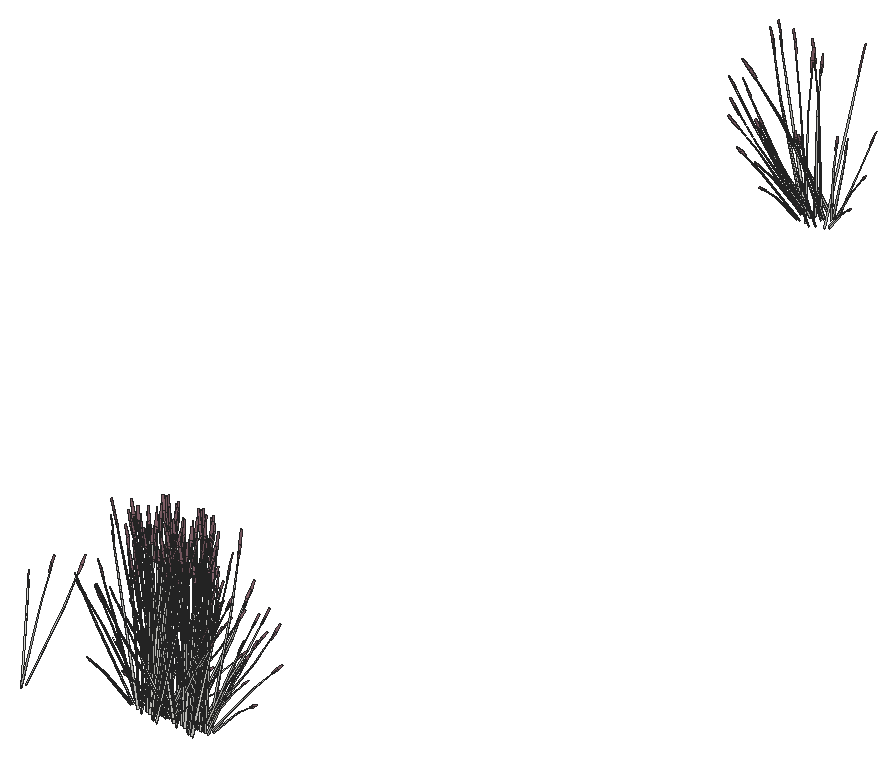
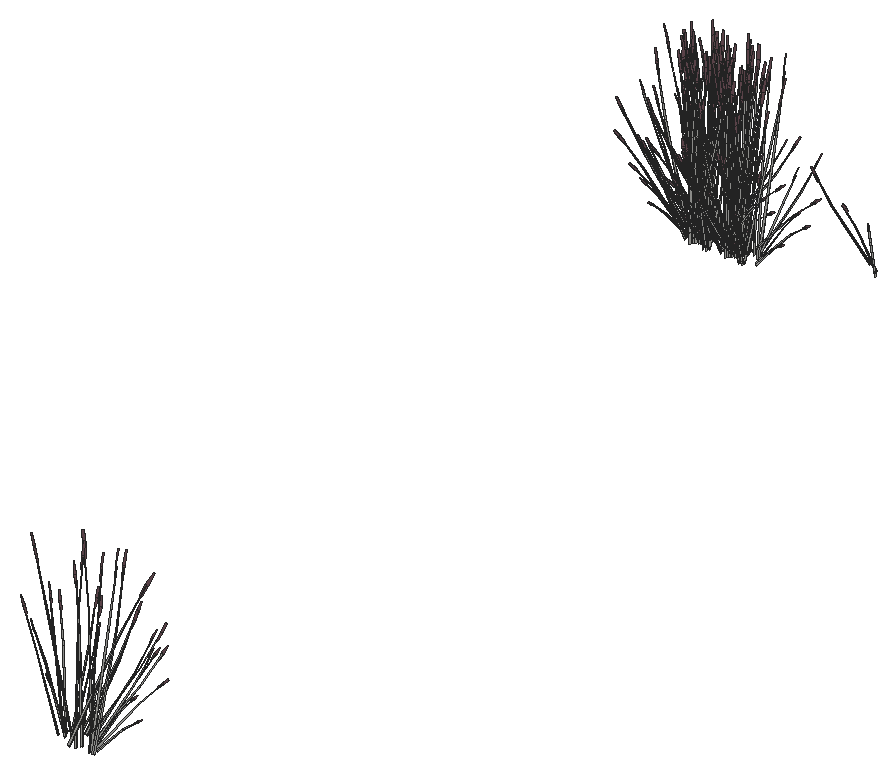
# SketchUp Ruby script. Lengths in inches.
U = 1.inch
M = Sketchup.active_model
def pt(a) = Geom::Point3d.new(a.map { |v| v * U })
def face(e, loops, mat)
  f = e.add_face(loops[0].map { |a| pt(a) })
  loops[1..].each { |l| e.add_face(l.map { |a| pt(a) }).erase! }
  f.material = f.back_material = mat if mat
  f
end
# faces: each face lists its corners as indices into pts; further lists are holes
def faces(e, pts, list, mat = nil) = list.each { |f| face(e, (f[0].is_a?(Array) ? f : [f]).map { |l| l.map { |i| pts[i] } }, mat) }
# xy, xz, yz: faces in a plane at the given z, y or x. An outline is a flat list of corners, or four numbers for a rectangle; further outlines are holes
def ring(l) = l.size == 4 ? [[l[0], l[1]], [l[2], l[1]], [l[2], l[3]], [l[0], l[3]]] : l.each_slice(2).to_a
def flat(e, list, mat, &to3) = list.each { |f| face(e, (f[0].is_a?(Array) ? f : [f]).map { |l| ring(l).map { |u, v| to3.(u, v) } }, mat) }
def xy(e, z, list, mat = nil) = flat(e, list, mat) { |x, y| [x, y, z] }
def xz(e, y, list, mat = nil) = flat(e, list, mat) { |x, z| [x, y, z] }
def yz(e, x, list, mat = nil) = flat(e, list, mat) { |y, z| [x, y, z] }
def lines(e, pts, list) = list.each { |a, b| e.add_line(pt(pts[a]), pt(pts[b])) }
# prism: a flat outline (further loops are holes) pulled along v
def prism(e, loops, v, mat = nil)
  f = face(e, loops, mat); d = Geom::Vector3d.new(v.map { |x| x * U })
  f.pushpull(f.normal.samedirection?(d) ? d.length : -d.length)
end
def box(e, o, s, mat = nil) = prism(e, [[o, [o[0] + s[0], o[1], o[2]], [o[0] + s[0], o[1] + s[1], o[2]], [o[0], o[1] + s[1], o[2]]]], [0, 0, s[2]], mat)
def at(x, y, z, deg = 0) = Geom::Transformation.translation(pt([x, y, z])) * Geom::Transformation.rotation(ORIGIN, Z_AXIS, deg.degrees)
def axes(o, x, y, z) = Geom::Transformation.new([*x, 0, *y, 0, *z, 0, *pt(o).to_a, 1])
def part(name) = M.definitions.add(name)
# library, detail: a bought-in or finely detailed component or shape, given as its bounding box
def library(name, o, s) = part(name).tap { |d| box(d.entities, o, s) }
def detail(e, o, s) = box(e.add_group.entities, o, s)
def put(e, d, t, mat = nil) = e.add_instance(d, t).tap { |i| i.material = mat if mat }
def group(e, t, mat = nil) = e.add_group.tap { |g| g.transformation = t; g.material = mat if mat }.entities
root = M.entities
M.materials.add("LightPink_Translucent").color = [144, 107, 117]
c1 = part("blade")
p = [[2.15,0.21,22],[0,0.17,0],[0.09,0.45,0],[2.18,0.31,22],[2.29,0.31,22],[0.38,0.45,0],
  [2.48,0.24,33],[2.49,0.24,33],[2.48,0.22,33]]
faces(c1.entities,p,[[0,1,2,3],[4,5,2,3],[6,3,4,7],[8,0,3,6]])
c2 = part("seeds")
p = [[0.3,-0.1,1.38],[-0.01,-0.03,1.59],[-0.01,-0.03,0.03],[0.14,-0.07,-0.07],[0.29,-0.03,3],[0.15,0.01,3.11]]
faces(c2.entities,p,[[0,1,2,3],[1,0,4,5]],"LightPink_Translucent")
c3 = part("blade with seeds")
put(c3.entities,c1,at(0,0,0))
put(c3.entities,c2,axes([2.4,0.25,30.99],[1.5799,-0.05474,1.17369],[-0.12525,1.92788,0.29478],[-0.07173,-0.02425,1.56792]))
put(root,c3,axes([71.27,71.75,46.98],[-1.22504,-0.02494,-0.71045],[0.08228,-1.05005,0.08574],[-0.51899,-0.11081,1.00501]))
put(root,c3,axes([30.98,61.23,46.98],[0.5849,0.8421,-0.71045],[-1.20401,0.4693,0.08574],[0.13677,0.40688,1.00501]))
put(root,c3,axes([27.6,62.55,44.59],[0.38672,-0.16338,1.43002],[0.95481,0.49262,-0.30754],[-0.28419,0.42626,0.61141]))
put(root,c3,axes([59.21,73.76,44.33],[-1.1399,0.87071,0.30756],[-1.1406,-0.86155,-0.36492],[-0.03981,-0.24727,1.64885]))
put(root,c3,axes([71.21,73.76,44.33],[-1.1399,0.87071,0.30756],[-1.1406,-0.86155,-0.36492],[-0.03981,-0.24727,1.64885]))
put(root,c3,axes([62.84,74.17,44.43],[1.3808,0.50196,0.24065],[-0.66454,1.04299,0.50002],[0,-0.24043,1.60543]))
put(root,c3,axes([74.84,74.17,44.43],[1.3808,0.50196,0.24065],[-0.66454,1.04299,0.50002],[0,-0.24043,1.60543]))
put(root,c3,axes([58.87,71.96,46.68],[-0.88986,0.68603,-0.51099],[-0.77932,-0.72471,-0.3958],[-0.45212,-0.10438,0.97773]))
put(root,c3,axes([70.87,71.96,46.68],[-0.88986,0.68603,-0.51099],[-0.77932,-0.72471,-0.3958],[-0.45212,-0.10438,0.97773]))
put(root,c3,axes([56.86,72.87,44.77],[0.78239,-0.07411,1.1486],[-0.49629,0.65296,0.84392],[-0.38663,-0.09795,0.25299]))
put(root,c3,axes([68.86,72.87,44.77],[0.78239,-0.07411,1.1486],[-0.49629,0.65296,0.84392],[-0.38663,-0.09795,0.25299]))
put(root,c3,axes([28.1,61.75,45.36],[0.02693,-0.53464,1.54345],[1.21102,0.2824,0.21329],[-0.10493,0.5698,0.72882]))
put(root,c3,axes([62.39,73.47,44.72],[-1.33077,0.06393,0.44739],[-0.12035,-1.06125,-0.21531],[0.23824,-0.10756,1.43643]))
put(root,c3,axes([74.39,73.47,44.72],[-1.33077,0.06393,0.44739],[-0.12035,-1.06125,-0.21531],[0.23824,-0.10756,1.43643]))
put(root,c3,axes([58.95,74.25,44.48],[0,1.03566,0.49651],[-1.37109,0,0],[0,-0.23588,1.57504]))
put(root,c3,axes([70.95,74.25,44.48],[0,1.03566,0.49651],[-1.37109,0,0],[0,-0.23588,1.57504]))
put(root,c3,axes([68.58,74.48,46.68],[0.332,-0.94205,-0.51099],[1.13828,0.3229,-0.3958],[0.45829,-0.08638,0.97773]))
put(root,c3,axes([80.58,74.48,46.68],[0.332,-0.94205,-0.51099],[1.13828,0.3229,-0.3958],[0.45829,-0.08638,0.97773]))
put(root,c3,axes([66.78,70.64,44.375],[0.7662,-1.03778,0],[1.28187,0.57875,-0.51607],[0.29196,0.13181,1.63711]))
put(root,c3,axes([78.78,70.64,44.375],[0.7662,-1.03778,0],[1.28187,0.57875,-0.51607],[0.29196,0.13181,1.63711]))
put(root,c3,axes([62.34,73.85,44.36],[0.53281,1.15808,0.45755],[-1.52239,0.4027,0.17955],[0.01861,-0.2128,1.58856]))
put(root,c3,axes([74.34,73.85,44.36],[0.53281,1.15808,0.45755],[-1.52239,0.4027,0.17955],[0.01861,-0.2128,1.58856]))
put(root,c3,axes([69.79,74.74,43.98],[-0.7893,0.12429,1.41583],[-0.12563,-0.9893,0.08104],[0.55282,-0.14974,0.80566]))
put(root,c3,axes([81.79,74.74,43.98],[-0.7893,0.12429,1.41583],[-0.12563,-0.9893,0.08104],[0.55282,-0.14974,0.80566]))
put(root,c3,axes([62.08,74.77,44.72],[-0.59459,0.93321,0.44739],[-1.23546,-0.44912,-0.21531],[0,-0.21512,1.43643]))
put(root,c3,axes([74.08,74.77,44.72],[-0.59459,0.93321,0.44739],[-1.23546,-0.44912,-0.21531],[0,-0.21512,1.43643]))
put(root,c3,axes([64.26,73.95,44.21],[0,-1.19833,0],[1.53239,0,0],[0,0,1.79456]))
put(root,c3,axes([76.26,73.95,44.21],[0,-1.19833,0],[1.53239,0,0],[0,0,1.79456]))
put(root,c3,axes([66.12,71.18,44.48],[-1.14694,-0.51783,0.49651],[0.68554,-0.92854,0],[0.26122,0.11794,1.57504]))
put(root,c3,axes([78.12,71.18,44.48],[-1.14694,-0.51783,0.49651],[0.68554,-0.92854,0],[0.26122,0.11794,1.57504]))
put(root,c3,axes([68.36,74.82,46.98],[1.07686,-0.45739,-0.71045],[0.60013,0.94154,0.08574],[0.52031,-0.10696,1.00501]))
put(root,c3,axes([80.36,74.82,46.98],[1.07686,-0.45739,-0.71045],[0.60013,0.94154,0.08574],[0.52031,-0.10696,1.00501]))
put(root,c3,axes([63.53,73.2,44.36],[-1.01611,0.93987,0.45755],[-1.20717,-0.82966,0.17955],[0.24496,-0.0938,1.58856]))
put(root,c3,axes([75.53,73.2,44.36],[-1.01611,0.93987,0.45755],[-1.20717,-0.82966,0.17955],[0.24496,-0.0938,1.58856]))
put(root,c3,axes([64.64,74.88,44.3],[-1.1399,-0.8914,-0.06131],[1.1406,-0.89194,0],[-0.03981,-0.03113,1.75571]))
put(root,c3,axes([76.64,74.88,44.3],[-1.1399,-0.8914,-0.06131],[1.1406,-0.89194,0],[-0.03981,-0.03113,1.75571]))
put(root,c3,axes([61.77,71.65,44.47],[-0.35402,1.02926,0.17642],[-1.29548,-0.29127,0.35086],[0.22379,-0.00501,1.60407]))
put(root,c3,axes([73.77,71.65,44.47],[-0.35402,1.02926,0.17642],[-1.29548,-0.29127,0.35086],[0.22379,-0.00501,1.60407]))
put(root,c3,axes([64.48,72.79,44.62],[0.23642,-0.92427,0.1448],[1.15506,0.16044,-0.41347],[0.21021,0.09491,1.26744]))
put(root,c3,axes([76.48,72.79,44.62],[0.23642,-0.92427,0.1448],[1.15506,0.16044,-0.41347],[0.21021,0.09491,1.26744]))
put(root,c3,axes([62.48,74.99,44.36],[1.54892,0.2182,0.45755],[-0.31522,1.23236,0.17955],[-0.22636,-0.119,1.58856]))
put(root,c3,axes([74.48,74.99,44.36],[1.54892,0.2182,0.45755],[-0.31522,1.23236,0.17955],[-0.22636,-0.119,1.58856]))
put(root,c3,axes([63.98,73.04,44.72],[-0.73619,-0.86927,0.44739],[1.11511,-0.61213,-0.21531],[0.23824,0.10756,1.43643]))
put(root,c3,axes([75.98,73.04,44.72],[-0.73619,-0.86927,0.44739],[1.11511,-0.61213,-0.21531],[0.23824,0.10756,1.43643]))
put(root,c3,axes([61.65,76.96,44.47],[1.31687,-0.27488,0.17642],[0.32517,1.02297,0.35086],[-0.11745,-0.14905,1.60407]))
put(root,c3,axes([73.65,76.96,44.47],[1.31687,-0.27488,0.17642],[0.32517,1.02297,0.35086],[-0.11745,-0.14905,1.60407]))
put(root,c3,axes([65.3,74.22,44.21],[1.37109,0,0],[0,1.07219,0],[0,0,1.78407]))
put(root,c3,axes([77.3,74.22,44.21],[1.37109,0,0],[0,1.07219,0],[0,0,1.78407]))
put(root,c3,axes([65.6875,71.7,44.47],[-1.31687,0.27488,0.17642],[-0.32517,-1.02297,0.35086],[0.11745,0.14905,1.60407]))
put(root,c3,axes([77.6875,71.7,44.47],[-1.31687,0.27488,0.17642],[-0.32517,-1.02297,0.35086],[0.11745,0.14905,1.60407]))
put(root,c3,axes([64.86,73.67,44.38],[-1.54892,-0.2182,0.49198],[0.31522,-1.23236,0.19306],[0.22636,0.119,1.70813]))
put(root,c3,axes([76.86,73.67,44.38],[-1.54892,-0.2182,0.49198],[0.31522,-1.23236,0.19306],[0.22636,0.119,1.70813]))
put(root,c3,axes([63.62,76.72,44.2],[-0.39985,-0.89288,0],[1.1418,-0.31268,0],[0,0,1.54371]))
put(root,c3,axes([75.62,76.72,44.2],[-0.39985,-0.89288,0],[1.1418,-0.31268,0],[0,0,1.54371]))
put(root,c3,axes([62.86,75.87,44.62],[-0.23642,0.92427,0.1448],[-1.15506,-0.16044,-0.41347],[-0.21021,-0.09491,1.26744]))
put(root,c3,axes([74.86,75.87,44.62],[-0.23642,0.92427,0.1448],[-1.15506,-0.16044,-0.41347],[-0.21021,-0.09491,1.26744]))
put(root,c3,axes([65.5625,77.01,44.47],[0.35402,-1.02926,0.17642],[1.29548,0.29127,0.35086],[-0.22379,0.00501,1.60407]))
put(root,c3,axes([77.5625,77.01,44.47],[0.35402,-1.02926,0.17642],[1.29548,0.29127,0.35086],[-0.22379,0.00501,1.60407]))
put(root,c3,axes([65.27,74.68,44.21],[0.85545,0.66896,0],[-0.85545,0.66896,0],[0,0,1.69266]))
put(root,c3,axes([77.27,74.68,44.21],[0.85545,0.66896,0],[-0.85545,0.66896,0],[0,0,1.69266]))
put(root,c3,axes([60.41,73.42,45.34],[0.34834,-0.14982,1.77064],[0.12012,1.04605,0.13857],[-0.75452,0.1388,0.63284]))
put(root,c3,axes([72.41,73.42,45.34],[0.34834,-0.14982,1.77064],[0.12012,1.04605,0.13857],[-0.75452,0.1388,0.63284]))
put(root,c3,axes([67.59,74.39,44.47],[-0.96285,-0.75439,0.17642],[0.97031,-0.7317,0.35086],[-0.10634,0.15406,1.60407]))
put(root,c3,axes([79.59,74.39,44.47],[-0.96285,-0.75439,0.17642],[0.97031,-0.7317,0.35086],[-0.10634,0.15406,1.60407]))
put(root,c3,axes([71.4375,75.08,44.77],[-0.75718,0.17097,1.1486],[0.35641,-0.70661,0.84392],[0.40168,0.04835,0.25299]))
put(root,c3,axes([83.4375,75.08,44.77],[-0.75718,0.17097,1.1486],[0.35641,-0.70661,0.84392],[0.40168,0.04835,0.25299]))
put(root,c3,axes([63.34,77.12,44.2],[-1.23546,-0.46496,0],[0.59459,-0.96613,0],[0,0,1.62707]))
put(root,c3,axes([75.34,77.12,44.2],[-1.23546,-0.46496,0],[0.59459,-0.96613,0],[0,0,1.62707]))
put(root,c3,axes([61.22,77.48,44.48],[1.14694,0.51783,0.49651],[-0.68554,0.92854,0],[-0.26122,-0.11794,1.57504]))
put(root,c3,axes([73.22,77.48,44.48],[1.14694,0.51783,0.49651],[-0.68554,0.92854,0],[-0.26122,-0.11794,1.57504]))
put(root,c3,axes([65.26,73.9,44.72],[0.59459,-0.93321,0.44739],[1.23546,0.44912,-0.21531],[0,0.21512,1.43643]))
put(root,c3,axes([77.26,73.9,44.72],[0.59459,-0.93321,0.44739],[1.23546,0.44912,-0.21531],[0,0.21512,1.43643]))
put(root,c3,axes([65.03,74.43,44.29],[0,1.19774,-0.05637],[-1.53239,0,0],[0,0.03764,1.79368]))
put(root,c3,axes([77.03,74.43,44.29],[0,1.19774,-0.05637],[-1.53239,0,0],[0,0.03764,1.79368]))
put(root,c3,axes([58,73.99,46.68],[-0.332,0.94205,-0.51099],[-1.13828,-0.3229,-0.3958],[-0.45829,0.08638,0.97773]))
put(root,c3,axes([70,73.99,46.68],[-0.332,0.94205,-0.51099],[-1.13828,-0.3229,-0.3958],[-0.45829,0.08638,0.97773]))
put(root,c3,axes([60.56,78.02,44.375],[-0.7662,1.03778,0],[-1.28187,-0.57875,-0.51607],[-0.29196,-0.13181,1.63711]))
put(root,c3,axes([72.56,78.02,44.375],[-0.7662,1.03778,0],[-1.28187,-0.57875,-0.51607],[-0.29196,-0.13181,1.63711]))
put(root,c3,axes([68.38,74.42,44.48],[0,-1.03566,0.49651],[1.37109,0,0],[0,0.23588,1.57504]))
put(root,c3,axes([80.38,74.42,44.48],[0,-1.03566,0.49651],[1.37109,0,0],[0,0.23588,1.57504]))
put(root,c3,axes([64.94,75.19,44.72],[1.33077,-0.06393,0.44739],[0.12035,1.06125,-0.21531],[-0.23824,0.10756,1.43643]))
put(root,c3,axes([76.94,75.19,44.72],[1.33077,-0.06393,0.44739],[0.12035,1.06125,-0.21531],[-0.23824,0.10756,1.43643]))
put(root,c3,axes([65.77,74.11,44.62],[1.1418,-0.30203,0.1448],[0.39985,0.86246,-0.41347],[0,0.18981,1.26744]))
put(root,c3,axes([77.77,74.11,44.62],[1.1418,-0.30203,0.1448],[0.39985,0.86246,-0.41347],[0,0.18981,1.26744]))
put(root,c3,axes([70.02,76.21,44.59],[-0.29514,-0.25472,1.43002],[0.38401,-0.84262,-0.30754],[0.59714,0.11414,0.61141]))
put(root,c3,axes([82.02,76.21,44.59],[-0.29514,-0.25472,1.43002],[0.38401,-0.84262,-0.30754],[0.59714,0.11414,0.61141]))
put(root,c3,axes([64.74,77.14,44.2],[1.23546,0.46496,0],[-0.59459,0.96613,0],[0,0,1.74954]))
put(root,c3,axes([76.74,77.14,44.2],[1.23546,0.46496,0],[-0.59459,0.96613,0],[0,0,1.74954]))
put(root,c3,axes([65.23,78.17,44.19],[-0.75665,-1.04141,-0.05142],[1.28187,-0.57875,0.51607],[-0.31588,0.09915,1.6363]))
put(root,c3,axes([77.23,78.17,44.19],[-0.75665,-1.04141,-0.05142],[1.28187,-0.57875,0.51607],[-0.31588,0.09915,1.6363]))
put(root,c3,axes([64.97,75.65,44.62],[0.90538,0.62224,0.1448],[-0.75521,0.70202,-0.41347],[-0.21021,0.09491,1.26744]))
put(root,c3,axes([76.97,75.65,44.62],[0.90538,0.62224,0.1448],[-0.75521,0.70202,-0.41347],[-0.21021,0.09491,1.26744]))
put(root,c3,axes([67.31,76.72,46.98],[1.22504,0.02494,-0.71045],[-0.08228,1.05005,0.08574],[0.51899,0.11081,1.00501]))
put(root,c3,axes([79.31,76.72,46.98],[1.22504,0.02494,-0.71045],[-0.08228,1.05005,0.08574],[0.51899,0.11081,1.00501]))
put(root,c3,axes([65.93,77.56,44.48],[1.14694,-0.51783,0.49651],[0.68554,0.92854,0],[-0.26122,0.11794,1.57504]))
put(root,c3,axes([77.93,77.56,44.48],[1.14694,-0.51783,0.49651],[0.68554,0.92854,0],[-0.26122,0.11794,1.57504]))
put(root,c3,axes([64.3,76.75,44.29],[0.53281,1.18979,-0.06012],[-1.52239,0.41691,0],[0.01861,0.04155,1.72173]))
put(root,c3,axes([76.3,76.75,44.29],[0.53281,1.18979,-0.06012],[-1.52239,0.41691,0],[0.01861,0.04155,1.72173]))
put(root,c3,axes([56.64,76.2,44.59],[0.42589,0.08502,1.43002],[0.2745,0.86839,-0.30754],[-0.57851,0.16255,0.61141]))
put(root,c3,axes([68.64,76.2,44.59],[0.42589,0.08502,1.43002],[0.2745,0.86839,-0.30754],[-0.57851,0.16255,0.61141]))
put(root,c3,axes([69.31,74.59,44.375],[1.53239,0,0],[0,1.1575,-0.51607],[0,0.26363,1.63711]))
put(root,c3,axes([81.31,74.59,44.375],[1.53239,0,0],[0,1.1575,-0.51607],[0,0.26363,1.63711]))
put(root,c3,axes([68.7,75.1875,44.2],[-1.53164,-0.00828,-0.04976],[0,-1.1575,0.49943],[-0.04813,0.2635,1.58352]))
put(root,c3,axes([80.7,75.1875,44.2],[-1.53164,-0.00828,-0.04976],[0,-1.1575,0.49943],[-0.04813,0.2635,1.58352]))
put(root,c3,axes([55.75,78.02,44.77],[0.51072,-0.46938,1.1486],[0.20153,0.74307,0.84392],[-0.36908,0.13305,0.25299]))
put(root,c3,axes([67.75,78.02,44.77],[0.51072,-0.46938,1.1486],[0.20153,0.74307,0.84392],[-0.36908,0.13305,0.25299]))
put(root,c3,axes([65.27,77.63,44.33],[1.53422,0.33662,0.30756],[-0.38383,1.20322,-0.36492],[-0.25393,0.15059,1.64885]))
put(root,c3,axes([77.27,77.63,44.33],[1.53422,0.33662,0.30756],[-0.38383,1.20322,-0.36492],[-0.25393,0.15059,1.64885]))
put(root,c3,axes([67.23,77.53,44.77],[-0.69001,-0.29779,1.1486],[0.89096,-0.30257,0.84392],[0.24031,0.2563,0.25299]))
put(root,c3,axes([79.23,77.53,44.77],[-0.69001,-0.29779,1.1486],[0.89096,-0.30257,0.84392],[0.24031,0.2563,0.25299]))
put(root,c3,axes([58.56,76.09,46.68],[0.31482,0.94565,-0.51099],[-1.19224,0.16542,-0.3958],[-0.34166,0.254,0.97773]))
put(root,c3,axes([70.56,76.09,46.68],[0.31482,0.94565,-0.51099],[-1.19224,0.16542,-0.3958],[-0.34166,0.254,0.97773]))
put(root,c3,axes([66.2,78.28,44.375],[0.7662,1.03778,0],[-1.28187,0.57875,-0.51607],[-0.29196,0.13181,1.63711]))
put(root,c3,axes([78.2,78.28,44.375],[0.7662,1.03778,0],[-1.28187,0.57875,-0.51607],[-0.29196,0.13181,1.63711]))
put(root,c3,axes([65.55,74.17,44.84],[-0.03348,-0.97511,1.41272],[1.51511,0.25277,0.59816],[-0.35835,0.53357,1.3335]))
put(root,c3,axes([77.55,74.17,44.84],[-0.03348,-0.97511,1.41272],[1.51511,0.25277,0.59816],[-0.35835,0.53357,1.3335]))
put(root,c3,axes([65.67,77.9375,46.68],[1.20928,-0.24619,-0.51099],[0.21154,0.93233,-0.3958],[0.32481,0.26718,0.97773]))
put(root,c3,axes([77.67,77.9375,46.68],[1.20928,-0.24619,-0.51099],[0.21154,0.93233,-0.3958],[0.32481,0.26718,0.97773]))
put(root,c3,axes([67.34,78.88,44.67],[-0.78586,-0.03248,1.0506],[0.51898,-0.68985,0.58006],[0.31045,0.24509,0.8241]))
put(root,c3,axes([79.34,78.88,44.67],[-0.78586,-0.03248,1.0506],[0.51898,-0.68985,0.58006],[0.31045,0.24509,0.8241]))
put(root,c3,axes([64.77,77.21,44.59],[0.02163,-0.34331,1.43002],[1.03345,-0.38348,-0.30754],[0.31903,0.4109,0.61141]))
put(root,c3,axes([76.77,77.21,44.59],[0.02163,-0.34331,1.43002],[1.03345,-0.38348,-0.30754],[0.31903,0.4109,0.61141]))
put(root,c3,axes([60.08,80.07,44.77],[-0.03171,-0.6158,1.1486],[0.7925,0.43922,0.84392],[-0.15586,0.29352,0.25299]))
put(root,c3,axes([72.08,80.07,44.77],[-0.03171,-0.6158,1.1486],[0.7925,0.43922,0.84392],[-0.15586,0.29352,0.25299]))
put(root,c3,axes([60.38,77.69,47],[0.87728,0.69587,-0.5672],[-0.92674,0.60943,-0.43934],[-0.13348,0.35356,1.08528]))
put(root,c3,axes([72.38,77.69,47],[0.87728,0.69587,-0.5672],[-0.92674,0.60943,-0.43934],[-0.13348,0.35356,1.08528]))
put(root,c3,axes([59.43,78.74,44.82],[1.11329,-0.1834,0.06507],[0.25594,0.73887,-0.86304],[-0.07058,0.37403,0.7736]))
put(root,c3,axes([71.43,78.74,44.82],[1.11329,-0.1834,0.06507],[0.25594,0.73887,-0.86304],[-0.07058,0.37403,0.7736]))
put(root,c3,axes([62.98,78.37,46.68],[1.20468,0.25962,-0.51099],[-0.41292,0.89013,-0.3958],[0.11046,0.35838,0.97773]))
put(root,c3,axes([74.98,78.37,46.68],[1.20468,0.25962,-0.51099],[-0.41292,0.89013,-0.3958],[0.11046,0.35838,0.97773]))
put(root,c3,axes([60.11,77.375,47.34],[-0.03189,0.95798,-0.7886],[-1.34277,-0.06434,0.09517],[-0.14171,0.40585,1.11556]))
put(root,c3,axes([72.11,77.375,47.34],[-0.03189,0.95798,-0.7886],[-1.34277,-0.06434,0.09517],[-0.14171,0.40585,1.11556]))
put(root,c3,axes([62.54,78.2,46.98],[0.5849,0.8421,-0.71045],[-1.20401,0.4693,0.08574],[0.13677,0.40688,1.00501]))
put(root,c3,axes([74.54,78.2,46.98],[0.5849,0.8421,-0.71045],[-1.20401,0.4693,0.08574],[0.13677,0.40688,1.00501]))
put(root,c3,axes([59.16,79.52,44.59],[0.38672,-0.16338,1.43002],[0.95481,0.49262,-0.30754],[-0.28419,0.42626,0.61141]))
put(root,c3,axes([71.16,79.52,44.59],[0.38672,-0.16338,1.43002],[0.95481,0.49262,-0.30754],[-0.28419,0.42626,0.61141]))
put(root,c3,axes([59.66,78.73,45.36],[0.02693,-0.53464,1.54345],[1.21102,0.2824,0.21329],[-0.10493,0.5698,0.72882]))
put(root,c3,axes([71.66,78.73,45.36],[0.02693,-0.53464,1.54345],[1.21102,0.2824,0.21329],[-0.10493,0.5698,0.72882]))
put(root,c3,axes([36.79,388.28,44.59],[-0.34835,0.20963,1.43002],[-1.04325,-0.36691,-0.30754],[0.19338,-0.4563,0.61141]))
put(root,c3,axes([35.2,389.01,46.98],[-0.5849,-0.8421,-0.71045],[1.20401,-0.4693,0.08574],[-0.13677,-0.40688,1.00501]))
put(root,c3,axes([31.39,387.88,44.59],[-0.07421,0.33879,1.43002],[-1.08488,0.28361,-0.30754],[-0.25359,-0.4379,0.61141]))
put(root,c3,axes([37.63,389.83,46.98],[0.03189,-0.95798,-0.71045],[1.34277,0.06434,0.08574],[0.14171,-0.40585,1.00501]))
put(root,c3,axes([34.76,388.84,46.68],[-1.20468,-0.25962,-0.51099],[0.41292,-0.89013,-0.3958],[-0.11046,-0.35838,0.97773]))
put(root,c3,axes([35.5,386.61,44.77],[0.15721,0.60392,1.1486],[-0.87211,-0.33448,0.84392],[0.09385,-0.30923,0.25299]))
put(root,c3,axes([37.36,389.51,46.68],[-0.87728,-0.69587,-0.51099],[0.92674,-0.60943,-0.3958],[0.13348,-0.35356,0.97773]))
put(root,c3,axes([31.02,387.34,44.77],[0.63926,0.36046,1.1486],[-0.93099,0.21668,0.84392],[-0.1992,-0.27702,0.25299]))
put(root,c3,axes([32.5625,389.25,46.98],[-1.04497,-0.50058,-0.71045],[0.74264,-0.8772,0.08574],[-0.3786,-0.29889,1.00501]))
put(root,c3,axes([32.07,389.27,46.68],[-1.20928,0.24619,-0.51099],[-0.21154,-0.93233,-0.3958],[-0.32481,-0.26718,0.97773]))
put(root,c3,axes([39.22,391.5,46.98],[0.64013,-0.81717,-0.71045],[1.12174,0.58074,0.08574],[0.38221,-0.29607,1.00501]))
put(root,c3,axes([32.3,389.12,44.375],[-0.7662,-1.03778,0],[1.28187,-0.57875,-0.51607],[0.29196,-0.13181,1.63711]))
put(root,c3,axes([39.18,391.11,46.68],[-0.31482,-0.94565,-0.51099],[1.19224,-0.16542,-0.3958],[0.34166,-0.254,0.97773]))
put(root,c3,axes([35.0625,394.91,45.33],[1.05902,0.41762,1.51261],[-1.03748,0.89969,0.59816],[-0.46471,-0.53324,1.26806]))
put(root,c3,axes([40.14,390.75,44.59],[-0.4378,-0.03068,1.43002],[-0.44851,-0.8229,-0.30754],[0.53783,-0.23279,0.61141]))
put(root,c3,axes([40.65,389.23,44.77],[-0.40819,0.5272,1.1486],[-0.35086,-0.70831,0.84392],[0.33713,-0.17749,0.25299]))
put(root,c3,axes([29.18,392.81,44.375],[-1.53239,0,0],[0,-1.1575,-0.51607],[0,-0.26363,1.63711]))
put(root,c3,axes([29.44,390.74,44.59],[0.23927,0.28834,1.43002],[-0.55135,0.78376,-0.30754],[-0.56612,-0.18733,0.61141]))
put(root,c3,axes([30.43,390.48,46.98],[-1.22504,-0.02494,-0.71045],[0.08228,-1.05005,0.08574],[-0.51899,-0.11081,1.00501]))
put(root,c3,axes([30.37,392.5,44.33],[-1.1399,0.87071,0.30756],[-1.1406,-0.86155,-0.36492],[-0.03981,-0.24727,1.64885]))
put(root,c3,axes([34,392.91,44.43],[1.3808,0.50196,0.24065],[-0.66454,1.04299,0.50002],[0,-0.24043,1.60543]))
put(root,c3,axes([30.03,390.7,46.68],[-0.88986,0.68603,-0.51099],[-0.77932,-0.72471,-0.3958],[-0.45212,-0.10438,0.97773]))
put(root,c3,axes([28.02,391.61,44.77],[0.78239,-0.07411,1.1486],[-0.49629,0.65296,0.84392],[-0.38663,-0.09795,0.25299]))
put(root,c3,axes([33.55,392.21,44.72],[-1.33077,0.06393,0.44739],[-0.12035,-1.06125,-0.21531],[0.23824,-0.10756,1.43643]))
put(root,c3,axes([30.11,392.98,44.48],[0,1.03566,0.49651],[-1.37109,0,0],[0,-0.23588,1.57504]))
put(root,c3,axes([39.74,393.21,46.68],[0.332,-0.94205,-0.51099],[1.13828,0.3229,-0.3958],[0.45829,-0.08638,0.97773]))
put(root,c3,axes([37.9375,389.38,44.375],[0.7662,-1.03778,0],[1.28187,0.57875,-0.51607],[0.29196,0.13181,1.63711]))
